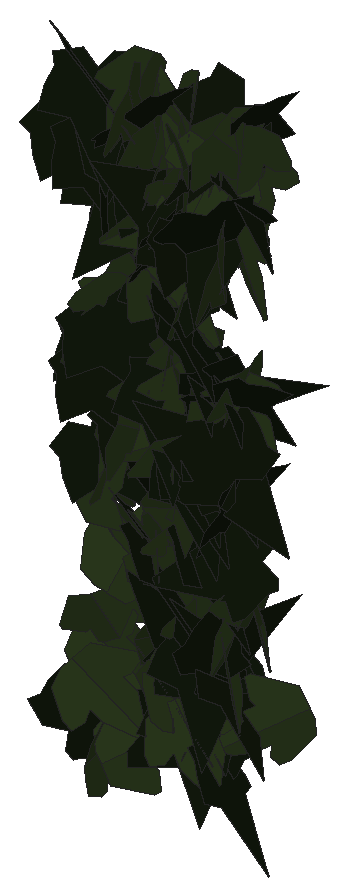
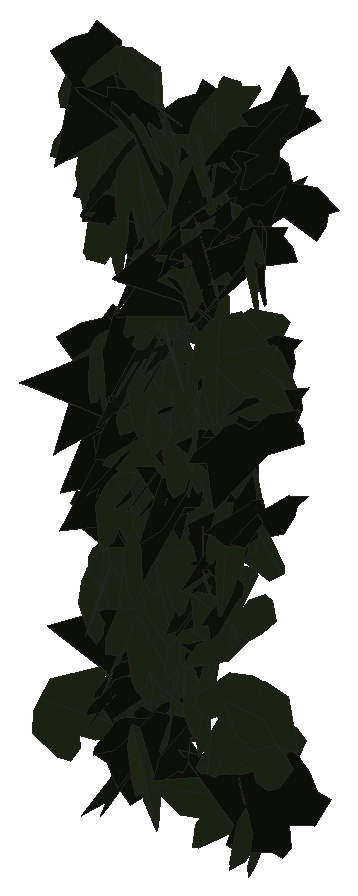
# SketchUp Ruby script. Lengths in inches.
U = 1.inch
M = Sketchup.active_model
def pt(a) = Geom::Point3d.new(a.map { |v| v * U })
def face(e, loops, mat)
  f = e.add_face(loops[0].map { |a| pt(a) })
  loops[1..].each { |l| e.add_face(l.map { |a| pt(a) }).erase! }
  f.material = f.back_material = mat if mat
  f
end
# faces: each face lists its corners as indices into pts; further lists are holes
def faces(e, pts, list, mat = nil) = list.each { |f| face(e, (f[0].is_a?(Array) ? f : [f]).map { |l| l.map { |i| pts[i] } }, mat) }
# xy, xz, yz: faces in a plane at the given z, y or x. An outline is a flat list of corners, or four numbers for a rectangle; further outlines are holes
def ring(l) = l.size == 4 ? [[l[0], l[1]], [l[2], l[1]], [l[2], l[3]], [l[0], l[3]]] : l.each_slice(2).to_a
def flat(e, list, mat, &to3) = list.each { |f| face(e, (f[0].is_a?(Array) ? f : [f]).map { |l| ring(l).map { |u, v| to3.(u, v) } }, mat) }
def xy(e, z, list, mat = nil) = flat(e, list, mat) { |x, y| [x, y, z] }
def xz(e, y, list, mat = nil) = flat(e, list, mat) { |x, z| [x, y, z] }
def yz(e, x, list, mat = nil) = flat(e, list, mat) { |y, z| [x, y, z] }
def lines(e, pts, list) = list.each { |a, b| e.add_line(pt(pts[a]), pt(pts[b])) }
# prism: a flat outline (further loops are holes) pulled along v
def prism(e, loops, v, mat = nil)
  f = face(e, loops, mat); d = Geom::Vector3d.new(v.map { |x| x * U })
  f.pushpull(f.normal.samedirection?(d) ? d.length : -d.length)
end
def box(e, o, s, mat = nil) = prism(e, [[o, [o[0] + s[0], o[1], o[2]], [o[0] + s[0], o[1] + s[1], o[2]], [o[0], o[1] + s[1], o[2]]]], [0, 0, s[2]], mat)
def at(x, y, z, deg = 0) = Geom::Transformation.translation(pt([x, y, z])) * Geom::Transformation.rotation(ORIGIN, Z_AXIS, deg.degrees)
def axes(o, x, y, z) = Geom::Transformation.new([*x, 0, *y, 0, *z, 0, *pt(o).to_a, 1])
def part(name) = M.definitions.add(name)
# library, detail: a bought-in or finely detailed component or shape, given as its bounding box
def library(name, o, s) = part(name).tap { |d| box(d.entities, o, s) }
def detail(e, o, s) = box(e.add_group.entities, o, s)
def put(e, d, t, mat = nil) = e.add_instance(d, t).tap { |i| i.material = mat if mat }
def group(e, t, mat = nil) = e.add_group.tap { |g| g.transformation = t; g.material = mat if mat }.entities
root = M.entities
M.materials.add("efeu1").color = [18, 25, 13]
M.materials.add("efeu2").color = [43, 57, 29]
c1 = part("ivyleaf_9")
p = [[1.54,2.16,1.25],[1.36,2.04,1.19],[-0.21,0.99,0.68],[-0.71,1.11,0.82],[-0.85,0.86,0.67],[-0.8,0.17,0.21],
  [-0.9,-0.01,0.1],[-0.67,-0.16,-0.02],[-0.08,-0.08,-0.05],[-0.03,-0.6,-0.4],[0.65,-0.88,-0.66],[0.83,-0.6,-0.49],
  [1.29,-0.42,-0.43],[1.8125,-0.07,-0.26],[1.21,0.44,0.15]]
faces(c1.entities,p,[[0,1,2,3,4,5,6,7,8,9,10,11,12,13,14]],"efeu1")
c2 = part("ivyleaf_10")
p = [[0,0.5,-0.03],[-0.0625,2.02,-0.43],[-0.19,2.01,-0.46],[-0.54,1.05,-0.29],[-0.52,0.625,-0.18],[-0.83,0.76,-0.28],
  [-1.16,0.64,-0.33],[-1.15,0.33,-0.24],[-0.77,-0.39,0.02],[-0.3,-0.51,0.16],[0.04,-0.48,0.23],[-0.02,2.01,-0.4375],
  [-0.06,2.01,-0.43],[0.04,-0.49,0.23],[0.67,-0.49,0.14],[1.38,0.36,-0.2],[1.375,0.51,-0.24],[0.81,0.65,-0.19],
  [0.62,0.59,-0.15],[0.6,1.09,-0.28],[0.5,1.23,-0.31]]
faces(c2.entities,p,[[0,1,2,3,4,5,6,7,8,9,10],[11,12,0,13,14,15,16,17,18,19,20]],"efeu2")
put(root,c1,axes([23.28,224.42,219.3125],[-0.01479,-0.43124,-0.25261],[0.01697,0.25214,-0.43144],[0.49949,-0.02133,0.00718]))
put(root,c1,axes([23.11,223.9,222.41],[-0.01017,-0.21863,-0.44955],[0.35449,0.31389,-0.16067],[0.35247,-0.32199,0.14862]))
put(root,c2,axes([23.39,224.22,215.66],[-0.44211,-0.14612,-0.18216],[0.16792,0.07212,-0.4654],[0.16229,-0.4727,-0.0147]))
put(root,c2,axes([23.64,223.78,213.86],[0.04993,0.04056,0.49585],[-0.26085,0.42648,-0.00862],[-0.42363,-0.25782,0.06375]))
put(root,c1,axes([23.15,223.9375,214.05],[0.0128,0.00928,0.49975],[0.49344,-0.07998,-0.01115],[0.07974,0.49347,-0.01121]))
put(root,c1,axes([23.15,224.06,223.06],[0.26324,-0.32446,0.27466],[0.18197,-0.20595,-0.4177],[0.38418,0.31986,0.00965]))
put(root,c1,axes([23.36,224.08,222.08],[0.10051,-0.44841,-0.19705],[-0.03113,0.1949,-0.4594],[0.4888,0.10461,0.01126]))
put(root,c2,axes([23.67,224.35,219.76],[-0.15038,-0.2285,0.41854],[-0.07714,-0.42142,-0.25779],[0.47057,-0.14211,0.09149]))
put(root,c2,axes([23.21,224.28,215.15],[0.23675,0.10605,0.42744],[0.40088,0.14904,-0.25901],[-0.18234,0.46534,-0.01446]))
put(root,c1,axes([23.76,223.7,221.18],[0.03057,-0.06127,0.49529],[-0.10892,0.48344,0.06653],[-0.48703,-0.11196,0.01621]))
put(root,c1,axes([23.37,224.08,218.09],[0.17193,-0.31987,-0.34369],[-0.01438,0.36225,-0.34434],[0.46929,0.12829,0.11536]))
put(root,c1,axes([23.5,223.98,223.03],[-0.0471,-0.48019,-0.13115],[-0.00605,0.13228,-0.48215],[0.49774,-0.04383,-0.01827]))
put(root,c2,axes([23.68,224.09,221.78],[0.38811,-0.28994,-0.12371],[-0.06563,0.11761,-0.48152],[0.30832,0.39,0.05323]))
put(root,c2,axes([23.81,223.97,220.11],[0.18929,0.34305,-0.31062],[-0.25824,-0.20019,-0.37846],[-0.38403,0.30371,0.10139]))
put(root,c2,axes([23.72,224.22,217.85],[0.02187,-0.46669,-0.1781],[0.02461,0.17906,-0.46619],[0.49891,0.01162,0.0308]))
put(root,c1,axes([23.54,224.39,221.73],[-0.13119,-0.40401,-0.26376],[0.11064,0.24086,-0.42396],[0.46963,-0.1696,0.0262]))
put(root,c2,axes([23.42,223.92,217.42],[0.35054,-0.18149,-0.3069],[0.28251,-0.12116,0.39434],[-0.21751,-0.44987,0.0176]))
put(root,c2,axes([23.73,224.39,220.36],[-0.06644,-0.49351,-0.04513],[0.08315,0.03378,-0.49188],[0.48854,-0.07287,0.07758]))
put(root,c1,axes([23.56,223.85,219.28],[0.10458,-0.36964,-0.32004],[-0.02859,0.3221,-0.38136],[0.4881,0.09807,0.04623]))
put(root,c2,axes([23.54,223.71,214.99],[0.25648,0.24595,0.35175],[0.23559,0.26185,-0.35487],[-0.35877,0.34777,0.01843]))
put(root,c2,axes([23.74,224.02,216.34],[0.25284,0.28745,-0.32163],[0.16528,0.27979,0.38],[0.39844,-0.29847,0.04646]))
put(root,c1,axes([23.94,224.33,221.38],[-0.30686,-0.35278,0.17716],[-0.0172,-0.21223,-0.4524],[0.39439,-0.28374,0.11811]))
put(root,c2,axes([23.95,224.26,223.09],[-0.04913,-0.4087,0.28381],[0.07299,-0.28803,-0.40213],[0.4922,0.00192,0.08797]))
put(root,c2,axes([24.3,224.08,216.7],[-0.25615,0.05127,-0.42633],[-0.4121,0.11015,0.26085],[0.12067,0.48501,-0.01417]))
put(root,c1,axes([23.77,223.82,219.96],[0.01687,-0.3356,-0.37025],[0.04657,0.36991,-0.33316],[0.49754,-0.02325,0.04374]))
put(root,c1,axes([23.72,224.2,217.17],[0.44226,-0.23292,0.01227],[0.01085,-0.00573,-0.49985],[0.233,0.44239,-0.00002]))
put(root,c1,axes([23.79,224.61,220.79],[0.11893,-0.46963,0.1237],[0.02264,-0.12186,-0.48439],[0.48512,0.12082,-0.00772]))
put(root,c2,axes([24.0625,224.375,221.82],[0.29183,-0.40582,0.01215],[0.00702,-0.00992,-0.49985],[0.40594,0.29191,-0.0001]))
put(root,c2,axes([24.15,224.37,218.87],[-0.10476,-0.44277,0.20733],[-0.01638,-0.20874,-0.45405],[0.48863,-0.10192,0.02923]))
put(root,c2,axes([24.11,224.28,222.32],[-0.05073,-0.46959,-0.16405],[0.04348,0.16009,-0.47168],[0.49552,-0.06212,0.02459]))
put(root,c2,axes([23.97,224.51,215.33],[0.03784,-0.20387,-0.45498],[0.06974,-0.44964,0.20728],[-0.49366,-0.07915,-0.00559]))
put(root,c1,axes([23.77,224.25,217.68],[0.0331,-0.18361,0.46389],[0.33752,-0.33412,-0.15633],[0.3674,0.3235,0.10182]))
put(root,c1,axes([24.13,223.73,222.69],[0.19705,0.42192,0.18208],[0.04286,0.18038,-0.46436],[-0.45753,0.19861,0.03492]))
put(root,c2,axes([24.04,224.0625,218.58],[-0.4266,-0.17014,-0.19765],[0.19823,0.03468,-0.45771],[0.16946,-0.46888,0.03786]))
put(root,c2,axes([24.17,223.71,223.04],[0.09523,-0.41134,-0.26783],[-0.00251,0.27241,-0.41927],[0.49084,0.0812,0.04982]))
put(root,c1,axes([23.98,224.16,218.68],[-0.00296,-0.23416,-0.44177],[0.0232,0.44124,-0.23403],[0.49945,-0.02188,0.00825]))
put(root,c1,axes([24.03,224.24,221.76],[0.16452,-0.36061,-0.30478],[-0.08575,0.29457,-0.39481],[0.46431,0.18218,0.03508]))
put(root,c2,axes([23.93,223.88,214.02],[0.15848,0.07097,-0.46888],[0.36629,0.29568,0.16855],[0.3012,-0.39691,0.04173]))
put(root,c2,axes([24.36,224.24,222.22],[0.43117,-0.06753,0.244],[-0.23715,0.06095,0.43594],[-0.08862,-0.49166,0.02053]))
put(root,c2,axes([24.26,223.54,218.73],[-0.00195,-0.28798,-0.40874],[0.07266,0.40424,-0.28515],[0.49469,-0.06051,0.04028]))
put(root,c2,axes([24.45,224.27,221.39],[0.01918,0.1023,-0.48905],[-0.28194,-0.40183,-0.09511],[-0.41248,0.27941,0.04227]))
put(root,c2,axes([24.35,224.26,218.97],[-0.40785,0.28668,0.03836],[-0.03383,0.01857,-0.49851],[-0.28725,-0.40923,0.00425]))
put(root,c2,axes([24.4375,224.29,221.22],[-0.4843,-0.11176,0.05448],[-0.05195,-0.01712,-0.497],[0.11295,-0.48705,0.00498]))
put(root,c2,axes([24.05,224.26,217.17],[0.17614,-0.12271,0.45157],[0.38779,-0.23178,-0.21424],[0.26191,0.4257,0.01352]))
put(root,c2,axes([24.42,224.5,220.79],[0.27431,0.32725,-0.26011],[-0.19525,-0.17479,-0.42582],[-0.36964,0.33519,0.03189]))
put(root,c2,axes([24.41,224.25,222.4375],[0.41291,-0.22558,-0.16916],[-0.09509,0.17099,-0.46013],[0.26545,0.41216,0.0983]))
put(root,c1,axes([24.52,224.23,221.28],[-0.02288,-0.49407,-0.07326],[0.01344,-0.07392,0.49432],[-0.4993,0.02065,0.01667]))
put(root,c1,axes([24.39,223.93,220.87],[0.18851,0.25835,0.38434],[0.14563,0.36085,-0.31398],[-0.43961,0.23032,0.0608]))
put(root,c1,axes([24.38,223.89,220.9375],[0.17622,0.14432,0.4451],[0.20582,0.40323,-0.21223],[-0.42022,0.25802,0.08271]))
put(root,c1,axes([24.21,224.01,216.88],[0.33543,-0.37079,-0.00112],[-0.00072,0.00086,-0.5],[0.3708,0.33543,0.00004]))
put(root,c2,axes([24.21,224.48,219.91],[-0.17908,0.11701,-0.45193],[0.35911,-0.27475,-0.21344],[-0.29828,-0.40103,0.01436]))
put(root,c2,axes([24.52,224.4,219.06],[0.06506,-0.42708,0.25173],[0.0293,-0.25014,-0.43194],[0.49488,0.07095,-0.00752]))
put(root,c2,axes([24.71,223.97,219.33],[-0.39921,0.17288,0.24647],[-0.23964,0.0653,-0.43395],[-0.18223,-0.46459,0.03072]))
put(root,c1,axes([24.89,224.24,220.59],[-0.41403,0.12978,0.24847],[-0.24263,0.05608,-0.43358],[-0.14041,-0.47959,0.01654]))
put(root,c2,axes([24.84,224.13,218.55],[-0.14138,-0.09122,0.47084],[-0.32945,-0.33825,-0.16446],[0.34853,-0.35674,0.03554]))
put(root,c2,axes([24.63,224.25,219.43],[-0.47738,-0.14545,0.03085],[-0.0288,-0.01131,-0.49904],[0.14587,-0.47824,0.00242]))
put(root,c2,axes([24.84,223.82,217.66],[0.21412,-0.07764,-0.44511],[-0.35227,0.27977,-0.21826],[0.28295,0.40707,0.06511]))
put(root,c2,axes([24.65,224.43,219.53],[-0.0557,-0.46246,0.18174],[-0.00441,-0.18242,-0.46552],[0.49687,-0.05346,0.01624]))
put(root,c2,axes([24.62,224.5625,216.26],[0.00198,-0.45694,0.20298],[0.0401,-0.20218,-0.45554],[0.49839,0.01808,0.03585]))
put(root,c2,axes([24.53,224.26,220.07],[0.27388,-0.3793,0.17641],[0.10975,-0.13832,-0.46778],[0.40366,0.29496,0.00749]))
put(root,c1,axes([24.625,224.18,218.39],[0.41021,0.06892,-0.27745],[-0.27154,-0.05783,-0.41584],[-0.08941,0.49184,-0.01002]))
put(root,c2,axes([24.71,224.35,217.09],[-0.17064,-0.46589,0.06186],[-0.02208,-0.05779,-0.49616],[0.46946,-0.17206,-0.00086]))
put(root,c2,axes([24.47,223.97,220.53],[-0.36342,-0.162,-0.30279],[0.31035,0.03377,-0.39057],[0.147,-0.47182,0.07601]))
put(root,c1,axes([24.76,224.17,218.92],[0.18864,0.37289,-0.27453],[-0.10584,-0.25387,-0.41755],[-0.45079,0.21565,-0.01685]))
put(root,c2,axes([24.75,223.77,214.92],[-0.03377,0.40224,-0.29507],[-0.05215,0.29128,0.40304],[0.49612,0.058,0.02228]))
put(root,c1,axes([24.52,224.1,219.1],[-0.02923,-0.49798,-0.03414],[0.00911,0.03366,-0.49878],[0.49906,-0.02978,0.0071]))
put(root,c2,axes([24.74,224.37,216.35],[-0.30474,-0.39587,-0.02047],[0.01334,0.01556,-0.49958],[0.39618,-0.30503,0.00108]))
put(root,c1,axes([24.35,224.2,214.87],[0.21895,-0.2998,0.33494],[0.19323,-0.27361,-0.37122],[0.40586,0.29199,-0.00395]))
put(root,c1,axes([25.01,224.26,214.625],[0.00408,0.03041,-0.49906],[-0.30726,-0.39356,-0.02649],[-0.39443,0.30689,0.01547]))
put(root,c2,axes([24.59,224.27,218.51],[0.30137,0.3824,0.1138],[0.04735,0.10733,-0.48604],[-0.39615,0.30373,0.02848]))
put(root,c2,axes([24.82,224.07,217.95],[-0.26525,0.42221,-0.03712],[-0.02314,0.02929,0.4986],[0.42321,0.26623,0.004]))
put(root,c2,axes([24.72,224.55,217.42],[0.02069,-0.44587,0.22533],[0.07433,-0.22026,-0.44267],[0.49401,0.05182,0.05717]))
put(root,c2,axes([24.46,224.34,217.3],[-0.30403,0.06247,-0.392],[0.37477,-0.11756,-0.3094],[-0.13082,-0.48195,0.02466]))
put(root,c2,axes([24.76,224.35,215.97],[0.06094,-0.4505,0.20818],[0.03716,-0.20501,-0.45452],[0.49488,0.07087,0.00849]))
put(root,c2,axes([24.64,224.3,223.02],[0.34288,-0.2936,0.21502],[0.1718,-0.12984,-0.45125],[0.32081,0.38333,0.01185]))
put(root,c2,axes([24.83,224.46,222.23],[-0.0356,-0.49679,0.04397],[0.01309,-0.04499,-0.4978],[0.49856,-0.03429,0.01621]))
put(root,c2,axes([24.89,224.14,219.25],[-0.26575,-0.3933,0.15715],[-0.03495,-0.16452,-0.47086],[0.42209,-0.26125,0.05995]))
put(root,c2,axes([24.97,224.125,216.76],[-0.45214,-0.14718,0.15461],[-0.13971,-0.06978,-0.47499],[0.1614,-0.47272,0.02198]))
put(root,c1,axes([24.51,224.24,220.15],[0.21382,-0.41373,0.18195],[0.09967,-0.15317,-0.46541],[0.44085,0.2353,0.01697]))
put(root,c2,axes([24.98,223.71,222.36],[0.22665,-0.17769,-0.40873],[-0.19527,0.3726,-0.27026],[0.40063,0.28213,0.0995]))
put(root,c2,axes([24.59,223.93,221.1],[0.40298,0.06603,-0.28853],[0.28514,0.04415,0.40834],[0.0794,-0.49365,-0.00207]))
put(root,c1,axes([25.09,223.97,215.58],[0.17927,-0.03782,0.46522],[-0.44453,0.13812,0.18252],[-0.14232,-0.47905,0.0159]))
put(root,c2,axes([24.9,224.38,214.61],[0.15334,-0.47589,-0.00394],[-0.00104,0.0038,-0.49998],[0.47591,0.15334,0.00018]))
put(root,c2,axes([24.63,223.92,215.41],[-0.25748,-0.11481,-0.41294],[0.38328,0.15392,-0.28178],[0.19183,-0.46166,0.00874]))
put(root,c2,axes([24.92,223.82,218.52],[-0.27906,-0.40464,-0.09161],[0.04131,0.08275,-0.49137],[0.41282,-0.28181,-0.01275]))
put(root,c1,axes([24.64,224.35,219.72],[0.14164,-0.4341,0.20371],[0.08046,-0.18789,-0.45632],[0.47272,0.16205,0.01663]))
put(root,c1,axes([24.8,223.88,221.44],[0.21966,-0.30197,-0.33251],[-0.17412,0.28395,-0.3729],[0.41404,0.27962,0.01959]))
put(root,c1,axes([24.75,224.07,218.28],[0.23458,-0.43074,-0.09713],[-0.04735,0.08481,-0.49047],[0.43901,0.23931,-0.00101]))
put(root,c1,axes([25.25,223.8,222.5],[-0.11898,0.42422,0.2364],[-0.11499,0.21186,-0.43806],[-0.47183,-0.15861,0.04714]))
put(root,c1,axes([24.83,224.08,218.21],[0.11654,-0.48211,-0.06319],[-0.01269,0.06194,-0.49599],[0.48606,0.11721,0.0022]))
put(root,c1,axes([24.88,224.38,215.49],[-0.03691,-0.47418,-0.15425],[0.01733,0.15336,-0.47559],[0.49833,-0.04045,0.00511]))
put(root,c1,axes([24.93,224.22,214.87],[-0.13083,-0.46951,-0.11153],[0.02316,0.10932,-0.48735],[0.48202,-0.13269,-0.00685]))
put(root,c2,axes([25.06,224.49,217.93],[-0.10409,-0.43175,0.22969],[0.06028,-0.24438,-0.43203],[0.48532,-0.06225,0.10293]))
put(root,c2,axes([25.13,224.25,221.86],[0.33819,-0.321,-0.18052],[-0.08837,0.16721,-0.46285],[0.35752,0.34497,0.05636]))
put(root,c1,axes([24.83,224.17,217.05],[0.30618,-0.3915,-0.05457],[-0.02564,0.0492,-0.49691],[0.39445,0.30709,0.01005]))
put(root,c2,axes([25.1,224.2,222.57],[0.39605,-0.30455,-0.01968],[-0.00908,0.02048,-0.4995],[0.30505,0.39601,0.01069]))
put(root,c1,axes([25.02,224.19,215.64],[-0.06487,-0.49518,-0.02423],[0.00316,0.02403,-0.49941],[0.49576,-0.06494,0.00001]))
put(root,c1,axes([25.1,224.28,221.61],[-0.3145,-0.35689,-0.15401],[0.11437,0.10438,-0.47542],[0.3715,-0.33427,0.01598]))
put(root,c2,axes([24.95,223.76,214.86],[0.36439,0.25851,0.22449],[0.17335,0.14341,-0.44652],[-0.29525,0.40325,0.01489]))
put(root,c1,axes([24.96,224.39,218.49],[0.17316,-0.4503,-0.13133],[-0.0229,0.13171,-0.4818],[0.4685,0.17288,0.02499]))
put(root,c1,axes([25.3,224.43,222.96],[-0.46474,-0.16937,-0.073],[0.06625,0.0314,-0.4946],[0.17212,-0.46939,-0.00674]))
put(root,c2,axes([25.24,224.11,222.47],[0.46923,0.08537,-0.15012],[-0.14805,-0.02493,-0.47693],[-0.08892,0.49203,0.00188]))
put(root,c1,axes([24.92,224.54,219.49],[0.16584,-0.39537,0.25726],[0.08743,-0.2422,-0.42859],[0.46352,0.18714,-0.0112]))
put(root,c1,axes([25.57,223.92,218.33],[-0.00597,0.05641,0.49677],[-0.49848,0.03755,-0.01026],[-0.03847,-0.49539,0.05579]))
put(root,c1,axes([25.35,223.74,221.82],[0.16586,0.4492,-0.14391],[-0.0539,-0.1335,-0.47882],[-0.4686,0.17435,0.00413]))
put(root,c1,axes([25.13,224.36,215.42],[0.22255,-0.44773,0.00261],[0.00468,-0.00059,-0.49998],[0.44771,0.22257,0.00393]))
put(root,c1,axes([25.45,223.92,217.8],[-0.11131,0.23625,-0.42637],[-0.23906,0.35469,0.25894],[0.42481,0.2615,0.03399]))
put(root,c1,axes([25.22,223.86,215.62],[0.04441,0.04622,0.49587],[0.37456,0.32501,-0.06384],[-0.32823,0.37714,-0.00576]))
put(root,c1,axes([25.09,224.02,219.15],[0.26047,0.06957,0.42109],[0.39345,0.15202,-0.26849],[-0.16539,0.47122,0.02445]))
put(root,c2,axes([25.33,224.16,215.79],[-0.20462,0.42614,-0.1629],[0.07146,-0.14639,-0.47272],[-0.45058,-0.21674,-0.001]))
put(root,c1,axes([25.8,224.11,217.16],[-0.42582,0.03796,0.2593],[-0.25995,0.00158,-0.42711],[-0.03325,-0.49855,0.01839]))
put(root,c1,axes([25.2,224.09,214.22],[0.31013,-0.39056,-0.03577],[-0.02328,0.02719,-0.49872],[0.39151,0.311,-0.00132]))
put(root,c2,axes([25.51,224.24,219.46],[0.06079,-0.49458,-0.04121],[-0.00037,0.04147,-0.49828],[0.49629,0.06061,0.00468]))
put(root,c2,axes([25.54,223.66,221.27],[0.13475,-0.39235,-0.27911],[-0.03393,0.28138,-0.41192],[0.4803,0.12995,0.0492]))
put(root,c1,axes([25.21,224.39,222.18],[0.24687,-0.41462,0.13095],[0.06777,-0.11205,-0.48255],[0.42949,0.256,0.00087]))
put(root,c2,axes([25.55,224.31,216.48],[0.03643,-0.42289,0.26426],[0.02236,-0.26332,-0.42446],[0.49817,0.04274,-0.00028]))
put(root,c2,axes([25.54,224.22,222.36],[-0.42325,-0.25827,-0.06447],[0.07266,0.0044,-0.49467],[0.25609,-0.42811,0.03381]))
put(root,c1,axes([25.4,223.87,219.34],[0.40388,0.28844,0.0607],[0.04765,0.03772,-0.49629],[-0.29088,0.40667,0.00298]))
put(root,c1,axes([25.27,224.02,218.41],[-0.08358,-0.17765,-0.45984],[0.2959,0.35496,-0.19092],[0.39428,-0.30404,0.0458]))
put(root,c2,axes([25.42,224.02,219.27],[-0.33703,-0.26706,-0.25512],[0.24043,0.10352,-0.426],[0.28036,-0.40983,0.05864]))
put(root,c2,axes([25.4,224.29,221.34],[-0.35874,0.19939,-0.28557],[0.20956,-0.20388,-0.40561],[-0.27819,-0.4107,0.06272]))
put(root,c2,axes([25.75,223.96,222.95],[-0.46177,-0.15605,0.11144],[-0.10256,-0.04455,-0.48734],[0.16202,-0.47293,0.00913]))
put(root,c2,axes([25.52,224.35,216.61],[-0.27527,0.38826,-0.15323],[0.0988,-0.11773,-0.47579],[-0.40554,-0.29222,-0.01191]))
put(root,c1,axes([25.63,223.88,222.99],[0.1791,0.41305,0.21752],[0.07892,0.20284,-0.45014],[-0.4601,0.19557,0.00746]))
put(root,c2,axes([25.57,223.76,222.93],[-0.16171,-0.33179,-0.33729],[0.17634,0.2885,-0.36834],[0.43904,-0.23809,0.02371]))
put(root,c2,axes([25.89,224.61,214.87],[-0.14748,-0.11474,0.46377],[-0.22271,-0.41289,-0.17297],[0.42267,-0.25759,0.07068]))
